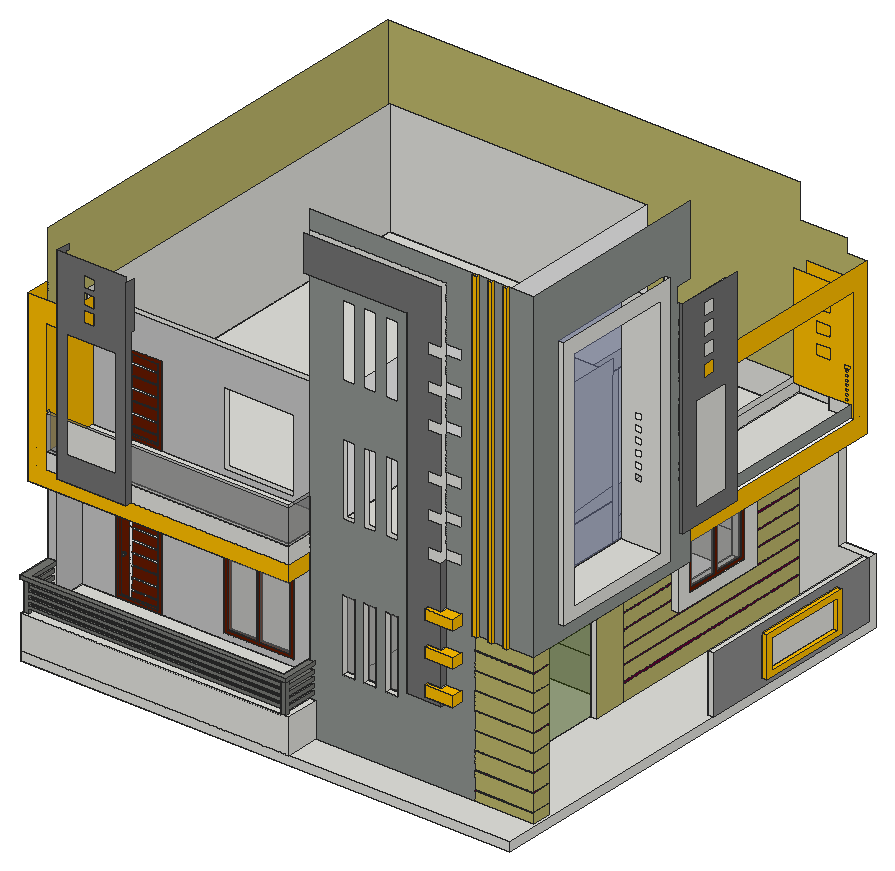
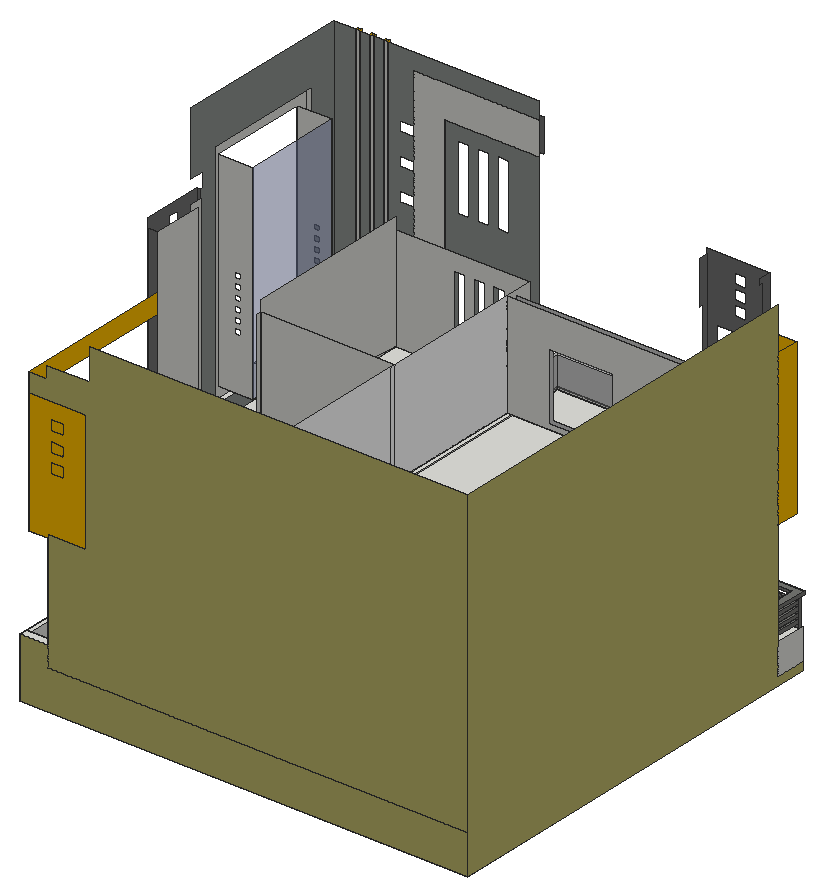
# SketchUp Ruby script. Lengths in inches.
U = 1.inch
M = Sketchup.active_model
def pt(a) = Geom::Point3d.new(a.map { |v| v * U })
def face(e, loops, mat)
  f = e.add_face(loops[0].map { |a| pt(a) })
  loops[1..].each { |l| e.add_face(l.map { |a| pt(a) }).erase! }
  f.material = f.back_material = mat if mat
  f
end
# faces: each face lists its corners as indices into pts; further lists are holes
def faces(e, pts, list, mat = nil) = list.each { |f| face(e, (f[0].is_a?(Array) ? f : [f]).map { |l| l.map { |i| pts[i] } }, mat) }
# xy, xz, yz: faces in a plane at the given z, y or x. An outline is a flat list of corners, or four numbers for a rectangle; further outlines are holes
def ring(l) = l.size == 4 ? [[l[0], l[1]], [l[2], l[1]], [l[2], l[3]], [l[0], l[3]]] : l.each_slice(2).to_a
def flat(e, list, mat, &to3) = list.each { |f| face(e, (f[0].is_a?(Array) ? f : [f]).map { |l| ring(l).map { |u, v| to3.(u, v) } }, mat) }
def xy(e, z, list, mat = nil) = flat(e, list, mat) { |x, y| [x, y, z] }
def xz(e, y, list, mat = nil) = flat(e, list, mat) { |x, z| [x, y, z] }
def yz(e, x, list, mat = nil) = flat(e, list, mat) { |y, z| [x, y, z] }
def lines(e, pts, list) = list.each { |a, b| e.add_line(pt(pts[a]), pt(pts[b])) }
# prism: a flat outline (further loops are holes) pulled along v
def prism(e, loops, v, mat = nil)
  f = face(e, loops, mat); d = Geom::Vector3d.new(v.map { |x| x * U })
  f.pushpull(f.normal.samedirection?(d) ? d.length : -d.length)
end
def box(e, o, s, mat = nil) = prism(e, [[o, [o[0] + s[0], o[1], o[2]], [o[0] + s[0], o[1] + s[1], o[2]], [o[0], o[1] + s[1], o[2]]]], [0, 0, s[2]], mat)
def at(x, y, z, deg = 0) = Geom::Transformation.translation(pt([x, y, z])) * Geom::Transformation.rotation(ORIGIN, Z_AXIS, deg.degrees)
def axes(o, x, y, z) = Geom::Transformation.new([*x, 0, *y, 0, *z, 0, *pt(o).to_a, 1])
def part(name) = M.definitions.add(name)
# library, detail: a bought-in or finely detailed component or shape, given as its bounding box
def library(name, o, s) = part(name).tap { |d| box(d.entities, o, s) }
def detail(e, o, s) = box(e.add_group.entities, o, s)
def put(e, d, t, mat = nil) = e.add_instance(d, t).tap { |i| i.material = mat if mat }
def group(e, t, mat = nil) = e.add_group.tap { |g| g.transformation = t; g.material = mat if mat }.entities
root = M.entities
M.materials.add("[0057_DarkKhaki]").color = [189, 183, 107]
M.materials.add("[Color B08]").color = [102, 25, 0]
M.materials.add("[Color D05]").color = [255, 191, 0]
M.materials.add("[Color L16]").color = [102, 0, 51]
M.materials.add("[Color M00]").color = [255, 255, 255]
M.materials.add("[Color M02]").color = [198, 198, 198]
M.materials.add("[Color M04]").color = [142, 142, 142]
M.materials.add("[Color M05]").color = [114, 114, 114]
M.materials.add("[Granite Light Gray]").color = [143, 148, 144]
M.materials.add("[Metal Seamed]").color = [118, 119, 115]
M.materials.add("[Translucent Glass Dark Green]").color = [62, 91, 5]
M.materials["[Translucent Glass Dark Green]"].alpha = 0.5
M.materials.add("[Translucent Glass Gray]").color = [128, 128, 128]
M.materials["[Translucent Glass Gray]"].alpha = 0.5
M.materials.add("[Translucent Glass Sky Reflection]").color = [126, 138, 183]
M.materials["[Translucent Glass Sky Reflection]"].alpha = 0.52
c1 = part("Group\#1")
xy(c1.entities,0,[[0,0,48,3.0625]],"[Color B08]")
xy(c1.entities,3.38,[[3.38,0,12.79,3.0625],[12.79,0,14.23,3.0625],[14.23,0,44.62,3.0625]],"[Color B08]")
xy(c1.entities,80.62,[[3.38,0,12.79,3.0625],[12.79,0,14.23,3.0625],[14.23,0,44.62,3.0625]],"[Color B08]")
xy(c1.entities,84,[[0,0,48,3.0625]],"[Color B08]")
xz(c1.entities,0,[[[0,0,48,84],[3.38,3.38,44.62,80.62]]],"[Color B08]")
xz(c1.entities,1.4375,[[7.15,41.24,7.55,41.32,7.92,41.49,8.23,41.75,8.46,42.09,8.6,42.47,8.63,42.88,8.5625,43.28,8.39,43.65,8.125,43.96,7.79,44.19,7.4,44.33,7,44.37,6.6,44.29,6.23,44.12,5.92,43.86,5.68,43.52,5.55,43.14,5.51,42.73,5.59,42.33,5.76,41.96,6.02,41.65,6.36,41.42,6.74,41.28]],"[Metal Seamed]")
xz(c1.entities,3.0625,[[14.23,33.6,44.62,34.93]])
xz(c1.entities,3.0625,[[[0,0,48,84],[3.38,3.38,44.62,80.62]],[[3.38,3.38,12.79,80.62],[7.15,41.24,6.74,41.28,6.36,41.42,6.02,41.65,5.76,41.96,5.59,42.33,5.51,42.73,5.55,43.14,5.68,43.52,5.92,43.86,6.23,44.12,6.6,44.29,7,44.37,7.4,44.33,7.79,44.19,8.125,43.96,8.39,43.65,8.5625,43.28,8.63,42.88,8.6,42.47,8.46,42.09,8.23,41.75,7.92,41.49,7.55,41.32]],[14.23,3.38,44.62,10.1],[14.23,11.43,44.62,21.85],[14.23,23.18,44.62,33.6],
  [14.23,34.93,44.62,45.35],[14.23,46.68,44.62,57.1],[14.23,58.43,44.62,68.85],[14.23,70.18,44.62,80.62]],"[Color B08]")
xz(c1.entities,3.0625,[[12.79,3.38,14.23,3.38,14.23,10.1,44.62,10.1,44.62,11.43,14.23,11.43,14.23,21.85,44.62,21.85,44.62,23.18,14.23,23.18,14.23,45.35,44.62,45.35,44.62,46.68,14.23,46.68,14.23,57.1,44.62,57.1,44.62,58.43,14.23,58.43,14.23,68.85,44.62,68.85,44.62,70.18,14.23,70.18,14.23,80.62,12.79,80.62]],"[Color M00]")
xz(c1.entities,3.0625,[[7.15,41.24,6.74,41.28,6.36,41.42,6.02,41.65,5.76,41.96,5.59,42.33,5.51,42.73,5.55,43.14,5.68,43.52,5.92,43.86,6.23,44.12,6.6,44.29,7,44.37,7.4,44.33,7.79,44.19,8.125,43.96,8.39,43.65,8.5625,43.28,8.63,42.88,8.6,42.47,8.46,42.09,8.23,41.75,7.92,41.49,7.55,41.32]],"[Metal Seamed]")
yz(c1.entities,0,[[0,0,3.0625,84]],"[Color B08]")
yz(c1.entities,3.38,[[0,3.38,3.0625,80.62]],"[Color B08]")
yz(c1.entities,44.62,[[0,3.38,3.0625,80.62]],"[Color B08]")
yz(c1.entities,48,[[0,0,3.0625,84]],"[Color B08]")
p = [[6.74,3.0625,41.28],[7.15,3.0625,41.24],[7.15,1.4375,41.24],[6.74,1.4375,41.28],[7.55,3.0625,41.32],[7.55,1.4375,41.32],
  [6.36,3.0625,41.42],[6.36,1.4375,41.42],[7.92,3.0625,41.49],[7.92,1.4375,41.49],[6.02,3.0625,41.65],[6.02,1.4375,41.65],
  [8.23,3.0625,41.75],[8.23,1.4375,41.75],[5.76,3.0625,41.96],[5.76,1.4375,41.96],[8.46,3.0625,42.09],[8.46,1.4375,42.09],
  [5.59,3.0625,42.33],[5.59,1.4375,42.33],[8.6,3.0625,42.47],[8.6,1.4375,42.47],[5.51,3.0625,42.73],[5.51,1.4375,42.73],
  [8.63,3.0625,42.88],[8.63,1.4375,42.88],[5.55,3.0625,43.14],[5.55,1.4375,43.14],[8.5625,3.0625,43.28],[8.5625,1.4375,43.28],
  [5.68,3.0625,43.52],[5.68,1.4375,43.52],[8.39,3.0625,43.65],[8.39,1.4375,43.65],[5.92,3.0625,43.86],[5.92,1.4375,43.86],
  [8.125,3.0625,43.96],[8.125,1.4375,43.96],[6.23,3.0625,44.12],[6.23,1.4375,44.12],[7.79,3.0625,44.19],[7.79,1.4375,44.19],
  [6.6,3.0625,44.29],[6.6,1.4375,44.29],[7.4,3.0625,44.33],[7.4,1.4375,44.33],[7,3.0625,44.37],[7,1.4375,44.37]]
faces(c1.entities,p,[[0,1,2,3],[1,4,5,2],[6,0,3,7],[4,8,9,5],[10,6,7,11],[8,12,13,9],[14,10,11,15],[12,16,17,13],
  [18,14,15,19],[16,20,21,17],[22,18,19,23],[20,24,25,21],[26,22,23,27],[24,28,29,25],[30,26,27,31],[28,32,33,29],
  [34,30,31,35],[32,36,37,33],[38,34,35,39],[36,40,41,37],[42,38,39,43],[40,44,45,41],[46,42,43,47],[44,46,47,45]],"[Metal Seamed]")
c2 = part("Group\#2")
xy(c2.entities,0,[[0,0,52.875,0.9375],[0,0.9375,52.875,3.1875]],"[Color B08]")
xy(c2.entities,2.82,[[2.82,0,24.76,0.9375],[26.4375,0,50.05,0.9375],[2.82,0.9375,24.76,3.1875],[26.4375,0.9375,50.05,3.1875]],"[Color B08]")
xy(c2.entities,69.3,[[2.82,0,24.76,0.9375],[26.4375,0,50.05,0.9375],[2.82,0.9375,24.76,3.1875],[26.4375,0.9375,50.05,3.1875]],"[Color B08]")
xy(c2.entities,72.125,[[0,0,52.875,0.9375],[0,0.9375,52.875,3.1875]],"[Color B08]")
xz(c2.entities,0,[[[0,0,52.875,72.125],[26.4375,2.82,50.05,69.3],[2.82,2.82,24.76,69.3]]],"[Color B08]")
xz(c2.entities,0.9375,[[[0,0,52.875,72.125],[26.4375,2.82,50.05,69.3],[2.82,2.82,24.76,69.3]]],"[Color B08]")
xz(c2.entities,0.9375,[[2.82,2.82,24.76,69.3],[26.4375,2.82,50.05,69.3]],"[Translucent Glass Gray]")
xz(c2.entities,3.1875,[[[0,0,52.875,72.125],[26.4375,2.82,50.05,69.3],[2.82,2.82,24.76,69.3]]],"[Color B08]")
yz(c2.entities,0,[[0,0,0.9375,72.125],[0.9375,0,3.1875,72.125]],"[Color B08]")
yz(c2.entities,2.82,[[0,2.82,0.9375,69.3],[0.9375,2.82,3.1875,69.3]],"[Color B08]")
yz(c2.entities,24.76,[[0,2.82,0.9375,69.3],[0.9375,2.82,3.1875,69.3]],"[Color B08]")
yz(c2.entities,26.4375,[[0,2.82,0.9375,69.3],[0.9375,2.82,3.1875,69.3]],"[Color B08]")
yz(c2.entities,50.05,[[0,2.82,0.9375,69.3],[0.9375,2.82,3.1875,69.3]],"[Color B08]")
yz(c2.entities,52.875,[[0,0,0.9375,72.125],[0.9375,0,3.1875,72.125]],"[Color B08]")
xy(root,0,[[0,1.9375,511.625,481.9375]])
xy(root,9,[[0,1.9375,0,37.27,9,37.27,9,10.9375,273.4375,10.9375,273.4375,38,279.9375,38,279.9375,1.9375],[279.9375,1.9375,511.625,1.9375,511.625,269.34,505.5625,269.34,505.5625,472.9375,438.3125,472.9375,438.3125,207.61,432.3125,207.61,432.3125,81.11,438.3125,81.11,438.3125,58.3125,508.125,58.3125,508.125,38,279.9375,38],[9,10.9375,273.0625,70.625],[273.0625,10.9375,273.4375,38],[9,76.625,273.0625,472.9375],
  [505.5625,269.34,511.625,472.9375]])
xy(root,9,[[279.0625,44,432.3125,236.875],[279.0625,236.875,432.3125,242.875],[279.0625,242.875,432.3125,472.9375]],"[Color M00]")
xy(root,18,[[511.625,332.96,516.8125,431.27]],"[Color D05]")
xy(root,23.63,[[511.625,338.58,516.8125,425.64]],"[Color D05]")
xy(root,45,[[[0,1.9375,272.41,1.9375,272.41,6.22,277.41,6.22,277.41,1.9375,279.9375,1.9375,279.9375,38,273.4375,38,273.4375,10.9375,9,10.9375,9,37.27,0,37.27],[0.99,3.54,6.11,6.22]],[9,10.9375,273.0625,70.625],[43.95,70.625,91.95,76.625]])
xy(root,45,[[272.41,1.9375,277.41,6.22],[0.99,3.54,6.11,6.22]],"[Metal Seamed]")
xy(root,49.55,[[6.11,3.54,274.92,6.22],[2.65,6.22,6.11,37.27],[272.41,6.22,274.92,38],[274.92,6.22,277.41,38]],"[Metal Seamed]")
xy(root,51.35,[[157.3,70.625,230.74,76.625]])
xy(root,53.05,[[6.11,3.54,274.92,6.22],[2.65,6.22,6.11,37.27],[272.41,6.22,274.92,38],[274.92,6.22,277.41,38]],"[Metal Seamed]")
xy(root,54.57,[[511.625,338.58,516.8125,425.64]],"[Color D05]")
xy(root,56.12,[[6.11,3.54,274.92,6.22],[2.65,6.22,6.11,37.27],[272.41,6.22,274.92,38],[274.92,6.22,277.41,38]],"[Metal Seamed]")
xy(root,59.62,[[6.11,3.54,274.92,6.22],[2.65,6.22,6.11,37.27],[272.41,6.22,274.92,38],[274.92,6.22,277.41,38]],"[Metal Seamed]")
xy(root,60.19,[[511.625,332.96,516.8125,431.27]],"[Color D05]")
xy(root,62.68,[[6.11,3.54,272.41,6.22],[2.65,6.22,6.11,37.27],[272.41,6.22,277.41,38.54]],"[Metal Seamed]")
xy(root,66.18,[[6.11,3.54,272.41,6.22],[2.65,6.22,6.11,37.27],[272.41,6.22,277.41,38.54]],"[Metal Seamed]")
xy(root,67.9,[[438.3125,305.17,446.125,407.29]])
xy(root,69,[[505.5625,269.34,511.625,472.9375],[480,472.9375,511.625,481.9375]])
xy(root,69.24,[[6.11,3.54,272.41,6.22],[2.65,6.22,6.11,37.27],[272.41,6.22,277.41,38]],"[Metal Seamed]")
xy(root,72.74,[[6.11,3.54,272.41,6.22],[2.65,6.22,6.11,37.27],[272.41,6.22,277.41,38]],"[Metal Seamed]")
xy(root,77.48,[[0,0,9,37.27],[9,0,9,6.22,272.41,6.22,272.41,1.9375,277.41,1.9375,277.41,6.22,271.72,6.22,271.72,70.625,278.6,70.625,278.6,0],[272.41,1.9375,277.41,6.22]],"[Metal Seamed]")
xy(root,78.125,[[0.99,3.54,6.11,6.22]],"[Metal Seamed]")
xy(root,78.97,[[307.95,38,320.7,44],[330.08,38,342.83,44],[353.14,38,365.89,44]])
xy(root,79.74,[[432.3125,318.89,446.125,392.02]])
xy(root,81,[[0,0,278.6,0,278.6,70.625,271.72,70.625,271.72,6.22,9,6.22,9,37.27,0,37.27]],"[Metal Seamed]")
xy(root,90.14,[[380.5625,31.1875,416.5625,38]],"[Color M05]")
xy(root,96.84,[[403.14,26.875,403.14,31.1875,416.5625,31.1875,416.5625,38,432.5625,38,432.5625,26.875]],"[Color D05]")
xy(root,107.44,[[403.14,26.875,432.5625,26.875,432.5625,38,416.5625,38,416.5625,31.1875,403.14,31.1875]],"[Color D05]")
xy(root,128.375,[[43.95,70.625,91.95,76.625]])
xy(root,128.41,[[157.3,70.625,230.74,76.625]])
xy(root,132.84,[[403.14,26.875,403.14,31.1875,416.5625,31.1875,416.5625,38.375,432.5625,38.375,432.5625,26.875]],"[Color D05]")
xy(root,143.44,[[403.14,26.875,432.5625,26.875,432.5625,38.375,416.5625,38.375,416.5625,31.1875,403.14,31.1875]],"[Color D05]")
xy(root,145.25,[[432.3125,81.11,438.3125,207.61]])
xy(root,147.99,[[432.3125,318.89,446.125,392.02]])
xy(root,154.03,[[307.95,38,320.7,44],[330.08,38,342.83,44],[353.14,38,365.89,44]])
xy(root,160.84,[[438.3125,305.17,446.125,407.29]])
xy(root,165,[[446.125,34.9375,450.58,38],[462.0625,34.9375,466.51,38],[478.1875,34.9375,482.64,38],[438.3125,58.3125,508.125,242.875]])
xy(root,165,[[0,10.9375,0,37.27,9,37.27,9,70.625,273.0625,70.625,273.0625,10.9375]],"[Color D05]")
xy(root,168.84,[[403.14,26.875,403.14,31.1875,416.5625,31.1875,416.5625,38,432.5625,38,432.5625,26.875]],"[Color D05]")
xy(root,178.3125,[[438.3125,242.875,438.3125,472.9375,480,472.9375,480,481.9375,502,481.9375,502,242.875]],"[Color D05]")
xy(root,179.44,[[403.14,26.875,432.5625,26.875,432.5625,38,416.5625,38,416.5625,31.1875,403.14,31.1875]],"[Color D05]")
xy(root,182,[[279.0625,242.875,432.3125,472.9375]])
xy(root,182,[[35.5,4.6875,107.76,10.9375]],"[Color M05]")
xy(root,183.33,[[508.125,69.42,515.125,208.18]])
xy(root,193,[[9,76.625,273.0625,472.9375]])
xy(root,196.21,[[474.9375,82.3,515.125,195.3]])
xy(root,198.0625,[[279.0625,44,432.3125,236.875]])
xy(root,199,[[19.8125,10.9375,19.8125,14.6875,270.25,14.6875,270.25,70.625,273.0625,70.625,273.0625,10.9375],[19.8125,14.6875,270.25,70.625],[279.0625,44,432.3125,236.875],[43.95,70.625,91.95,76.625],[9,76.625,273.0625,472.9375],
  [273.0625,76.625,279.0625,472.9375],[438.3125,242.875,438.3125,472.9375,475.75,472.9375,475.75,465.6875,498.1875,465.6875,498.1875,242.875],[500.3125,242.875,502,298.6875]])
xy(root,199,[[498.1875,242.875,498.1875,465.6875,502,465.6875,502,298.6875,500.3125,298.6875,500.3125,242.875]],"[Color M00]")
xy(root,199,[[508.125,228.57,508.125,242.875,502,242.875,502,298.6875,512.0625,298.6875,512.0625,228.57]],"[Color M05]")
xz(root,0,[[0,77.48,278.6,81]],"[Metal Seamed]")
xz(root,1.9375,[[0,0,511.625,9],[0,9,279.9375,45]])
xz(root,1.9375,[[272.41,45,277.41,77.48]],"[Metal Seamed]")
xz(root,3.54,[[0.99,45,6.11,45,6.11,49.55,274.92,49.55,274.92,53.05,6.11,53.05,6.11,56.12,274.92,56.12,274.92,59.62,6.11,59.62,6.11,62.68,272.41,62.68,272.41,66.18,6.11,66.18,6.11,78.125,0.99,78.125],[6.11,69.24,272.41,72.74]],"[Metal Seamed]")
xz(root,4.6875,[[[35.5,182,107.76,396.4375],[45.85,207.96,96.92,321.84],[63.1875,370.91,75.3125,383.04],[63.1875,354.54,75.3125,366.66],[63.1875,338.16,75.3125,350.29]]],"[Color M05]")
xz(root,6.22,[[0.99,45,0.99,78.125,6.11,78.125,6.11,72.74,2.65,72.74,2.65,69.24,6.11,69.24,6.11,66.18,2.65,66.18,2.65,62.68,6.11,62.68,6.11,59.62,2.65,59.62,2.65,56.12,6.11,56.12,6.11,53.05,2.65,53.05,2.65,49.55,6.11,49.55,6.11,45],[272.41,45,277.41,49.55],[2.65,49.55,6.11,53.05],[6.11,49.55,272.41,53.05],[272.41,53.05,277.41,56.12],
  [2.65,56.12,6.11,59.62],[6.11,56.12,272.41,59.62],[272.41,59.62,277.41,62.68],[2.65,62.68,6.11,66.18],[6.11,62.68,272.41,66.18],
  [272.41,66.18,277.41,69.24],[2.65,69.24,6.11,72.74],[6.11,69.24,272.41,72.74],[272.41,72.74,277.41,77.48],[9,77.48,271.72,81]],"[Metal Seamed]")
xz(root,10.9375,[[273.0625,9,273.4375,45],[19.8125,182,35.5,199],[35.5,182,107.76,199],[107.76,182,273.0625,199],[35.5,199,107.76,235]])
xz(root,10.9375,[[0,165,273.0625,165,273.0625,182,19.8125,182,19.8125,319,35.5,319,35.5,341.125,0,341.125]],"[Color D05]")
xz(root,10.9375,[[19.8125,199,35.5,235],[107.76,199,273.0625,235]],"[Translucent Glass Gray]")
xz(root,14.6875,[[19.8125,199,270.25,235]],"[Translucent Glass Gray]")
xz(root,26.875,[[403.14,96.84,432.5625,107.44],[403.14,132.84,432.5625,143.44],[403.14,168.84,432.5625,179.44]],"[Color D05]")
xz(root,31.1875,[[403.14,96.84,416.5625,107.44],[403.14,132.84,416.5625,143.44],[403.14,168.84,416.5625,179.44]])
xz(root,31.1875,[[380.5625,90.14,416.5625,90.14,416.5625,96.84,403.14,96.84,403.14,107.44,416.5625,107.44,416.5625,132.84,403.14,132.84,403.14,143.44,416.5625,143.44,416.5625,168.84,403.14,168.84,403.14,179.44,416.5625,179.44,416.5625,224.54,403.14,224.54,403.14,235.14,416.5625,235.14,416.5625,260.54,403.14,260.54,403.14,271.14,416.5625,271.14,416.5625,296.54,403.14,296.54,403.14,307.14,416.5625,307.14,416.5625,345.07,403.14,345.07,403.14,355.67,416.5625,355.67,416.5625,381.07,403.14,381.07,403.14,391.67,416.5625,391.67,416.5625,417.07,403.14,417.07,403.14,427.67,416.5625,427.67,416.5625,484.625,273.0625,484.625,273.0625,447.125,380.5625,447.125]],"[Color M05]")
xz(root,34.9375,[[446.125,165,450.58,504.125],[462.0625,165,466.51,504.125],[478.1875,165,482.64,504.125]],"[Color D05]")
xz(root,37.27,[[0,9,9,9,9,45,6.15,45,6.15,42.99,2.65,42.99,2.65,45,0,45],[2.65,42.99,6.15,45],[[0,45,9,77.48],[2.65,69.24,6.11,72.74],[2.65,62.68,6.11,66.18],[2.65,56.12,6.11,59.62],[2.65,49.55,6.11,53.05]],[0,165,9,182]])
xz(root,37.27,[[0,81,9,165]],"[Color M02]")
xz(root,37.27,[[2.65,49.55,6.11,53.05],[2.65,56.12,6.11,59.62],[2.65,62.68,6.11,66.18],[2.65,69.24,6.11,72.74],[0,77.48,9,81]],"[Metal Seamed]")
xz(root,38,[[273.0625,9,273.4375,45],[273.4375,9,279.9375,45],[380.5625,90.14,380.5625,447.125,273.0625,447.125,273.0625,484.625,416.5625,484.625,416.5625,90.14],[446.125,165,450.58,504.125],[462.0625,165,466.51,504.125],
  [478.1875,165,482.64,504.125]])
xz(root,38,[[446.125,9,508.125,18.7],[446.125,19.99,508.125,37.39],[446.125,38.68,508.125,56.07],[446.125,57.37,508.125,74.76],[446.125,76.05,508.125,93.45],
  [446.125,94.74,508.125,112.14],[446.125,113.43,508.125,130.82],[446.125,132.12,508.125,149.51],[446.125,150.8,508.125,165]],"[0057_DarkKhaki]")
xz(root,38,[[446.125,18.7,508.125,19.99],[446.125,37.39,508.125,38.68],[446.125,56.07,508.125,57.37],[446.125,74.76,508.125,76.05],[446.125,93.45,508.125,94.74],
  [446.125,112.14,508.125,113.43],[446.125,130.82,508.125,132.12],[446.125,149.51,508.125,150.8]],"[Color L16]")
xz(root,38,[[[279.9375,9,446.125,9,446.125,504.125,273.0625,504.125,273.0625,484.625,416.5625,484.625,416.5625,427.67,432.5625,427.67,432.5625,417.07,416.5625,417.07,416.5625,391.67,432.5625,391.67,432.5625,381.07,416.5625,381.07,416.5625,355.67,432.5625,355.67,432.5625,345.07,416.5625,345.07,416.5625,307.14,432.5625,307.14,432.5625,296.54,416.5625,296.54,416.5625,271.14,432.5625,271.14,432.5625,260.54,416.5625,260.54,416.5625,235.14,432.5625,235.14,432.5625,224.54,416.5625,224.54,416.5625,179.44,432.5625,179.44,432.5625,168.84,416.5625,168.84,416.5625,107.44,432.5625,107.44,432.5625,96.84,416.5625,96.84,416.5625,90.14,380.5625,90.14,380.5625,447.125,273.0625,447.125,273.0625,72.74,277.41,72.74,277.41,69.24,273.0625,69.24,273.0625,59.62,277.41,59.62,277.41,56.12,273.0625,56.12,273.0625,53.05,277.41,53.05,277.41,49.55,273.0625,49.55,273.0625,45,279.9375,45],[307.95,355.72,320.7,430.78],[330.08,355.72,342.83,430.78],[353.14,355.72,365.89,430.78],[307.95,224.97,320.7,300.03],[330.08,224.97,342.83,300.03],[353.14,224.97,365.89,300.03],[353.14,78.97,365.89,154.03],[330.08,78.97,342.83,154.03],[307.95,78.97,320.7,154.03]],[450.58,165,462.0625,504.125],[466.51,165,478.1875,504.125],[482.64,165,508.125,504.125]],"[Granite Light Gray]")
xz(root,38,[[272.41,49.55,273.0625,53.05],[273.0625,49.55,274.92,53.05],[272.41,56.12,273.0625,59.62],[273.0625,56.12,274.92,59.62],[272.41,69.24,273.0625,72.74],
  [273.0625,69.24,277.41,72.74]],"[Metal Seamed]")
xz(root,38.375,[[416.5625,132.84,432.5625,143.44]])
xz(root,38.54,[[272.41,62.68,277.41,66.18]],"[Metal Seamed]")
xz(root,44,[[279.0625,9,432.3125,45],[[279.0625,45,432.3125,165],[307.95,78.97,320.7,154.03],[330.08,78.97,342.83,154.03],[353.14,78.97,365.89,154.03]],[279.0625,165,432.3125,182],[279.0625,182,432.3125,198.0625],[279.0625,198.0625,325.8,199],
  [325.8,198.0625,340.67,199],[340.67,198.0625,432.3125,199],[[279.0625,199,432.3125,319],[307.95,224.97,320.7,300.03],[330.08,224.97,342.83,300.03],[353.14,224.97,365.89,300.03]]])
xz(root,44,[[307.95,78.97,320.7,154.03],[330.08,78.97,342.83,154.03],[353.14,78.97,365.89,154.03]],"[Translucent Glass Gray]")
xz(root,58.3125,[[438.3125,9,508.125,45],[438.3125,45,508.125,165]])
xz(root,69.42,[[508.125,183.33,515.125,449.28]])
xz(root,70.625,[[9,9,9,45,43.95,45,43.95,44.375,91.95,44.375,91.95,45,273.0625,45,273.0625,9],[43.95,44.375,91.95,45],[271.72,77.48,273.0625,81],[9,165,273.0625,182],[9,182,273.0625,199],
  [270.25,199,273.0625,235]])
xz(root,70.625,[[[9,45,43.95,45,43.95,128.375,91.95,128.375,91.95,45,273.0625,45,273.0625,77.48,271.72,77.48,271.72,81,273.0625,81,273.0625,165,9,165],[157.3,51.35,230.74,128.41]],[[19.8125,199,43.95,199,43.95,283,91.95,283,91.95,199,270.25,199,270.25,237.4375,273.0625,237.4375,273.0625,319,19.8125,319],[157.3,204.85,230.74,281.91]]],"[Color M02]")
xz(root,70.625,[[273.0625,77.48,278.6,81]],"[Metal Seamed]")
xz(root,76.625,[[9,9,273.0625,45],[[9,45,9,165,273.0625,165,273.0625,45,91.95,45,91.95,128.375,43.95,128.375,43.95,45],[157.3,51.35,230.74,128.41]],[9,165,273.0625,182],[9,182,273.0625,193],[9,193,43.95,199],
  [43.95,193,91.95,199],[91.95,193,248.5625,199],[248.5625,193,273.0625,199],[[9,199,9,319,279.0625,319,279.0625,199,91.95,199,91.95,283,43.95,283,43.95,199],[157.3,204.85,230.74,281.91]]])
xz(root,81.11,[[432.3125,9,438.3125,145.25]])
xz(root,82.3,[[[474.9375,196.21,515.125,433.9],[488.42,255.96,495.55,262.46],[488.42,267.52,495.55,274.02],[488.42,279.09,495.55,285.59],[488.42,290.65,495.55,297.15],[488.42,302.21,495.55,308.71],[488.42,313.77,495.55,320.27]]])
xz(root,195.3,[[[474.9375,196.21,515.125,433.9],[488.42,313.77,495.55,320.27],[488.42,302.21,495.55,308.71],[488.42,290.65,495.55,297.15],[488.42,279.09,495.55,285.59],[488.42,267.52,495.55,274.02],[488.42,255.96,495.55,262.46]]])
xz(root,207.61,[[432.3125,9,438.3125,145.25]])
xz(root,208.18,[[508.125,183.33,515.125,449.28]])
xz(root,228.57,[[508.125,199,512.0625,414.75]],"[Color M05]")
xz(root,236.875,[[279.0625,9,432.3125,45],[279.0625,45,432.3125,198.0625],[279.0625,198.0625,432.3125,199],[279.0625,199,432.3125,319]])
xz(root,242.875,[[279.0625,9,432.3125,45],[279.0625,45,432.3125,165],[279.0625,165,432.3125,182],[438.3125,165,508.125,178.3125],[438.3125,178.3125,502,199],
  [502,178.3125,508.125,199],[279.0625,182,432.3125,211],[438.3125,199,498.1875,211],[498.1875,199,500.3125,211],[500.3125,199,508.125,211]])
xz(root,269.34,[[505.5625,9,511.625,69]])
xz(root,298.6875,[[500.3125,199,512.0625,404.84]],"[Color M05]")
xz(root,305.17,[[438.3125,67.9,446.125,160.84]])
xz(root,318.89,[[432.3125,79.74,446.125,147.99]])
xz(root,332.96,[[511.625,18,516.8125,60.19]],"[Color D05]")
xz(root,338.58,[[511.625,23.63,516.8125,54.57]],"[Color D05]")
xz(root,392.02,[[432.3125,79.74,446.125,147.99]])
xz(root,407.29,[[438.3125,67.9,446.125,160.84]])
xz(root,425.64,[[511.625,23.63,516.8125,54.57]],"[Color D05]")
xz(root,431.27,[[511.625,18,516.8125,60.19]],"[Color D05]")
xz(root,465.6875,[[475.75,199,498.1875,211]])
xz(root,465.6875,[[[498.1875,199,502,199,502,319,438.3125,319,438.3125,211,490.625,211,490.625,247,497.9375,247,497.9375,243.89,490.625,243.89,490.625,211,498.1875,211],[462.25,289.25,477.19,301.1875],[462.25,266.5,477.19,278.4375],[462.25,245.375,477.19,257.3125],[492.23,213.64,496.17,216.08],[492.23,218.14,496.17,220.58],[492.23,222.64,496.17,225.08],[492.23,227.14,496.17,229.58],[492.23,231.64,496.17,234.08],[492.23,236.14,496.17,238.58],[492.23,240.26,496.17,242.7]]],"[Color D05]")
xz(root,472.9375,[[9,9,273.0625,45],[279.0625,9,432.3125,45],[438.3125,9,505.5625,9,505.5625,69,480,69,480,178.3125,438.3125,178.3125],[505.5625,9,511.625,69],[9,45,273.0625,165],
  [279.0625,45,432.3125,165],[9,165,273.0625,182],[279.0625,165,432.3125,182],[438.3125,178.3125,471,199],[471,178.3125,480,199],
  [9,182,273.0625,193],[279.0625,182,432.3125,211],[9,193,273.0625,199],[9,199,279.0625,319],[438.3125,199,471,211],
  [471,199,475.75,211]])
xz(root,481.9375,[[0,0,0,45,480,45,480,69,511.625,69,511.625,0],[0,45,0,390.75,432.3125,390.75,432.3125,354.75,481.39,354.75,481.39,341,502,341,502,319,438.3125,319,438.3125,182,480,182,480,45]],"[0057_DarkKhaki]")
xz(root,481.9375,[[[480,178.3125,480,182,438.3125,182,438.3125,319,502,319,502,178.3125],[462.25,245.375,477.19,257.3125],[462.25,266.5,477.19,278.4375],[462.25,289.25,477.19,301.1875]]],"[Color D05]")
yz(root,0,[[1.9375,9,37.27,45]])
yz(root,0,[[1.9375,0,1.9375,9,37.27,9,37.27,390.75,481.9375,390.75,481.9375,0]],"[0057_DarkKhaki]")
yz(root,0,[[10.9375,165,37.27,341.125]],"[Color D05]")
yz(root,0,[[0,77.48,37.27,81]],"[Metal Seamed]")
yz(root,0.99,[[3.54,45,6.22,78.125]],"[Metal Seamed]")
yz(root,2.65,[[6.22,49.55,37.27,53.05],[6.22,56.12,37.27,59.62],[6.22,62.68,37.27,66.18],[6.22,69.24,37.27,72.74]],"[Metal Seamed]")
yz(root,6.11,[[3.54,45,6.22,49.55],[6.22,49.55,37.27,53.05],[3.54,53.05,6.22,56.12],[6.22,56.12,37.27,59.62],[3.54,59.62,6.22,62.68],
  [6.22,62.68,37.27,66.18],[3.54,66.18,6.22,69.24],[3.54,69.24,6.22,72.74],[6.22,69.24,37.27,72.74],[3.54,72.74,6.22,78.125]],"[Metal Seamed]")
yz(root,9,[[10.9375,9,37.27,45],[37.27,9,70.625,45],[76.625,9,472.9375,45],[76.625,45,472.9375,165],[37.27,165,70.625,182],
  [76.625,165,472.9375,182],[76.625,182,472.9375,193],[76.625,193,472.9375,199],[76.625,199,472.9375,319]])
yz(root,9,[[37.27,45,70.625,165]],"[Color M02]")
yz(root,9,[[6.22,77.48,37.27,81]],"[Metal Seamed]")
yz(root,19.8125,[[10.9375,199,14.6875,235]])
yz(root,19.8125,[[14.6875,199,70.625,199,70.625,319,10.9375,319,10.9375,237.4375,14.6875,237.4375]],"[Color D05]")
yz(root,35.5,[[4.6875,182,4.6875,396.4375,19.25,396.4375,19.25,390.75,15.25,390.75,15.25,341.125,10.9375,341.125,10.9375,182]],"[Color M05]")
yz(root,43.95,[[70.625,45,76.625,128.375],[70.625,199,76.625,283]])
yz(root,91.95,[[70.625,45,76.625,128.375],[70.625,199,76.625,283]])
yz(root,107.76,[[4.6875,182,10.9375,182,10.9375,341.125,15.25,341.125,15.25,390.75,4.6875,390.75]],"[Color M05]")
yz(root,157.3,[[70.625,51.35,76.625,128.41]])
yz(root,230.74,[[70.625,51.35,76.625,128.41]])
yz(root,270.25,[[14.6875,199,70.625,235]],"[Translucent Glass Gray]")
yz(root,271.72,[[6.22,77.48,70.625,81]],"[Metal Seamed]")
yz(root,272.41,[[1.9375,45,1.9375,77.48,6.22,77.48,6.22,72.74,3.54,72.74,3.54,69.24,6.22,69.24,6.22,66.18,3.54,66.18,3.54,62.68,6.22,62.68,6.22,45],[6.22,49.55,38,53.05],[6.22,56.12,38,59.62],[3.54,62.68,6.22,66.18],[6.22,62.68,38.54,66.18],
  [3.54,69.24,6.22,72.74],[6.22,69.24,38,72.74]],"[Metal Seamed]")
yz(root,273.0625,[[10.9375,9,38,45],[38,9,70.625,45],[76.625,9,472.9375,45],[76.625,45,472.9375,165],[38,165,70.625,182],
  [76.625,165,472.9375,182],[10.9375,182,38,199],[38,182,70.625,199],[76.625,182,472.9375,193],[76.625,193,472.9375,199],
  [38,199,70.625,235]])
yz(root,273.0625,[[10.9375,165,38,182]],"[Color D05]")
yz(root,273.0625,[[38,45,70.625,165]],"[Granite Light Gray]")
yz(root,273.0625,[[10.9375,199,38,235]],"[Translucent Glass Gray]")
yz(root,273.4375,[[10.9375,9,38,45]])
yz(root,274.92,[[3.54,49.55,38,53.05],[3.54,56.12,38,59.62]],"[Metal Seamed]")
yz(root,277.41,[[1.9375,45,6.22,45,6.22,49.55,38,49.55,38,53.05,6.22,53.05,6.22,56.12,38,56.12,38,59.62,6.22,59.62,6.22,62.68,38.54,62.68,38.54,66.18,6.22,66.18,6.22,69.24,38,69.24,38,72.74,6.22,72.74,6.22,77.48,1.9375,77.48]],"[Metal Seamed]")
yz(root,278.6,[[0,77.48,70.625,81]],"[Metal Seamed]")
yz(root,279.0625,[[44,9,236.875,45],[236.875,9,242.875,45],[242.875,9,472.9375,45],[44,45,236.875,165],[236.875,45,242.875,165],
  [242.875,45,472.9375,165],[44,165,236.875,182],[236.875,165,242.875,182],[242.875,165,472.9375,182],[44,182,236.875,198.0625],
  [236.875,182,242.875,199],[242.875,182,472.9375,199],[44,198.0625,76.625,199],[76.625,198.0625,236.875,199],[44,199,76.625,319]])
yz(root,279.0625,[[76.625,199,236.875,319],[236.875,199,242.875,319],[242.875,199,472.9375,319]],"[Color M00]")
yz(root,279.9375,[[1.9375,9,38,45]])
yz(root,307.95,[[38,78.97,44,154.03]])
yz(root,320.7,[[38,78.97,44,154.03]])
yz(root,330.08,[[38,78.97,44,154.03]])
yz(root,342.83,[[38,78.97,44,154.03]])
yz(root,353.14,[[38,78.97,44,154.03]])
yz(root,365.89,[[38,78.97,44,154.03]])
yz(root,380.5625,[[31.1875,90.14,38,447.125]],"[Color M05]")
yz(root,403.14,[[26.875,96.84,31.1875,107.44],[26.875,132.84,31.1875,143.44],[26.875,168.84,31.1875,179.44]],"[Color D05]")
yz(root,416.5625,[[31.1875,96.84,38,107.44],[31.1875,132.84,38,143.44],[38,132.84,38.375,143.44],[31.1875,168.84,38,179.44]])
yz(root,416.5625,[[31.1875,90.14,38,96.84],[31.1875,107.44,38,132.84],[31.1875,143.44,38,168.84],[31.1875,179.44,38,224.54]],"[Color M05]")
yz(root,432.3125,[[44,9,81.11,45],[207.61,9,236.875,45],[236.875,9,242.875,319],[242.875,9,472.9375,45],[44,45,44,198.0625,236.875,198.0625,236.875,45,207.61,45,207.61,145.25,81.11,145.25,81.11,45],
  [[242.875,45,472.9375,165],[318.89,79.74,392.02,147.99]],[242.875,165,472.9375,182],[242.875,182,472.9375,211],[44,198.0625,236.875,199],[44,199,236.875,212.77,236.875,199],
  [44,199,44,331.875,236.875,331.875,236.875,212.77]])
yz(root,432.3125,[[81.11,9,207.61,145.25]],"[Translucent Glass Dark Green]")
yz(root,432.5625,[[26.875,96.84,38,107.44],[26.875,132.84,38.375,143.44],[26.875,168.84,38,179.44]],"[Color D05]")
yz(root,438.3125,[[305.17,75.66,407.29,77.77],[305.17,157.58,407.29,159.68],[242.875,178.3125,472.9375,199],[242.875,199,472.9375,211]])
yz(root,438.3125,[[58.3125,9,81.11,9,81.11,145.25,207.61,145.25,207.61,9,242.875,9,242.875,165,58.3125,165],[242.875,9,472.9375,26.51],[242.875,28.62,472.9375,42.89],[242.875,45,472.9375,59.28],[242.875,61.38,472.9375,61.38,472.9375,75.66,407.29,75.66,407.29,67.9,305.17,67.9,305.17,75.66,242.875,75.66],
  [242.875,77.77,305.17,92.04],[407.29,77.77,472.9375,92.04],[242.875,94.15,305.17,108.43],[407.29,94.15,472.9375,108.43],[242.875,110.53,305.17,124.81],
  [407.29,110.53,472.9375,124.81],[242.875,126.92,305.17,141.19],[407.29,126.92,472.9375,141.19],[242.875,143.3,305.17,157.58],[407.29,143.3,472.9375,157.58],
  [242.875,159.68,305.17,159.68,305.17,160.84,407.29,160.84,407.29,159.68,472.9375,159.68,472.9375,173.96,242.875,173.96],[242.875,176.07,472.9375,178.3125]],"[0057_DarkKhaki]")
yz(root,438.3125,[[242.875,26.51,472.9375,28.62],[242.875,42.89,472.9375,45],[242.875,59.28,472.9375,61.38],[242.875,75.66,305.17,77.77],[407.29,75.66,472.9375,77.77],
  [242.875,92.04,305.17,94.15],[407.29,92.04,472.9375,94.15],[242.875,108.43,305.17,110.53],[407.29,108.43,472.9375,110.53],[242.875,124.81,305.17,126.92],
  [407.29,124.81,472.9375,126.92],[242.875,141.19,305.17,143.3],[407.29,141.19,472.9375,143.3],[242.875,157.58,305.17,159.68],[407.29,157.58,472.9375,159.68],
  [242.875,173.96,472.9375,176.07]],"[Color L16]")
yz(root,446.125,[[[305.17,67.9,407.29,160.84],[318.89,79.74,392.02,147.99]]])
yz(root,446.125,[[34.9375,165,38,504.125]],"[Color D05]")
yz(root,450.58,[[34.9375,165,38,504.125]],"[Color D05]")
yz(root,462.0625,[[34.9375,165,38,504.125]],"[Color D05]")
yz(root,466.51,[[34.9375,165,38,504.125]],"[Color D05]")
yz(root,474.9375,[[82.3,196.21,195.3,433.9]],"[Translucent Glass Sky Reflection]")
yz(root,475.75,[[465.6875,199,472.9375,211]])
yz(root,478.1875,[[34.9375,165,38,504.125]],"[Color D05]")
yz(root,480,[[472.9375,69,481.9375,178.3125]])
yz(root,482.64,[[34.9375,165,38,504.125]],"[Color D05]")
yz(root,498.1875,[[242.875,199,465.6875,211]],"[Granite Light Gray]")
yz(root,500.3125,[[242.875,199,298.6875,404.84]])
yz(root,502,[[242.875,178.3125,481.9375,178.3125,481.9375,341,242.875,341,242.875,319,465.6875,319,465.6875,199,242.875,199]],"[Color D05]")
yz(root,505.5625,[[269.34,9,472.9375,69]])
yz(root,508.125,[[228.57,199,242.875,404.84]])
yz(root,508.125,[[38,9,58.3125,19.14],[38,20.43,58.3125,37.76],[38,39.05,58.3125,56.39],[38,57.68,58.3125,75.01],[38,76.3,58.3125,93.64],
  [38,94.93,58.3125,112.26],[38,113.55,58.3125,130.89],[38,132.18,58.3125,149.51],[38,150.8,58.3125,165]],"[0057_DarkKhaki]")
yz(root,508.125,[[38,19.14,58.3125,20.43],[38,37.76,58.3125,39.05],[38,56.39,58.3125,57.68],[38,75.01,58.3125,76.3],[38,93.64,58.3125,94.93],
  [38,112.26,58.3125,113.55],[38,130.89,58.3125,132.18],[38,149.51,58.3125,150.8]],"[Color L16]")
yz(root,508.125,[[[38,165,242.875,165,242.875,199,228.57,199,228.57,414.75,225.38,414.75,225.38,431.25,242.875,431.25,242.875,504.125,38,504.125],[69.42,183.33,208.18,449.28]]],"[Granite Light Gray]")
yz(root,511.625,[[1.9375,0,481.9375,0,481.9375,69,472.9375,69,472.9375,9,1.9375,9],[338.58,23.63,425.64,54.57]])
yz(root,511.625,[[[332.96,18,431.27,60.19],[338.58,23.63,425.64,54.57]]],"[Color D05]")
yz(root,511.625,[[[269.34,9,472.9375,69],[332.96,18,431.27,60.19]]],"[Color M04]")
yz(root,512.0625,[[[228.57,199,298.6875,414.75],[246.21,216.14,285.27,316.45],[256.47,390.6875,269.66,403.875],[256.47,371.4375,269.66,384.625],[256.47,352.1875,269.66,365.375],[256.47,332.9375,269.66,346.125]]],"[Color M05]")
yz(root,515.125,[[[69.42,183.33,208.18,449.28],[82.3,196.21,195.3,433.9]]])
yz(root,516.8125,[[[332.96,18,431.27,60.19],[338.58,23.63,425.64,54.57]]],"[Color D05]")
p = [[9,70.625,199],[9,10.9375,199],[9,37.27,182],[9,10.9375,182],[480,472.9375,199],[502,472.9375,199],
  [446.125,38,1.3],[446.125,38,0.01],[508.125,38,1.3],[508.125,38,0.01]]
lines(root,p,[[0,1],[2,3],[4,5],[6,7],[8,6],[9,8]])
put(root,c1,at(43.95,70.625,44.375),"[Color M02]")
put(root,c2,axes([157.3,70.625,51.35],[1.38889,0,0],[0,1.405,0],[0,0,1.06846]))
put(root,c2,axes([445.05,318.89,80.49],[0,1.41582,0],[-1.06833,0,0],[0,0,0.93592]))
put(root,c1,at(43.95,70.625,199))
